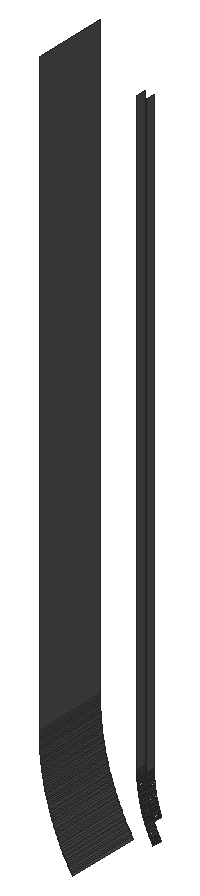
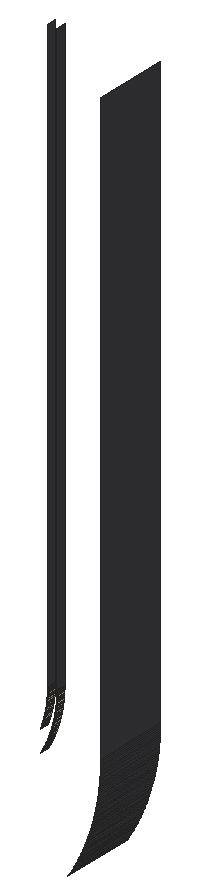
# SketchUp Ruby script. Lengths in inches.
U = 1.inch
M = Sketchup.active_model
def pt(a) = Geom::Point3d.new(a.map { |v| v * U })
def face(e, loops, mat)
  f = e.add_face(loops[0].map { |a| pt(a) })
  loops[1..].each { |l| e.add_face(l.map { |a| pt(a) }).erase! }
  f.material = f.back_material = mat if mat
  f
end
# faces: each face lists its corners as indices into pts; further lists are holes
def faces(e, pts, list, mat = nil) = list.each { |f| face(e, (f[0].is_a?(Array) ? f : [f]).map { |l| l.map { |i| pts[i] } }, mat) }
# xy, xz, yz: faces in a plane at the given z, y or x. An outline is a flat list of corners, or four numbers for a rectangle; further outlines are holes
def ring(l) = l.size == 4 ? [[l[0], l[1]], [l[2], l[1]], [l[2], l[3]], [l[0], l[3]]] : l.each_slice(2).to_a
def flat(e, list, mat, &to3) = list.each { |f| face(e, (f[0].is_a?(Array) ? f : [f]).map { |l| ring(l).map { |u, v| to3.(u, v) } }, mat) }
def xy(e, z, list, mat = nil) = flat(e, list, mat) { |x, y| [x, y, z] }
def xz(e, y, list, mat = nil) = flat(e, list, mat) { |x, z| [x, y, z] }
def yz(e, x, list, mat = nil) = flat(e, list, mat) { |y, z| [x, y, z] }
def lines(e, pts, list) = list.each { |a, b| e.add_line(pt(pts[a]), pt(pts[b])) }
# prism: a flat outline (further loops are holes) pulled along v
def prism(e, loops, v, mat = nil)
  f = face(e, loops, mat); d = Geom::Vector3d.new(v.map { |x| x * U })
  f.pushpull(f.normal.samedirection?(d) ? d.length : -d.length)
end
def box(e, o, s, mat = nil) = prism(e, [[o, [o[0] + s[0], o[1], o[2]], [o[0] + s[0], o[1] + s[1], o[2]], [o[0], o[1] + s[1], o[2]]]], [0, 0, s[2]], mat)
def at(x, y, z, deg = 0) = Geom::Transformation.translation(pt([x, y, z])) * Geom::Transformation.rotation(ORIGIN, Z_AXIS, deg.degrees)
def axes(o, x, y, z) = Geom::Transformation.new([*x, 0, *y, 0, *z, 0, *pt(o).to_a, 1])
def part(name) = M.definitions.add(name)
# library, detail: a bought-in or finely detailed component or shape, given as its bounding box
def library(name, o, s) = part(name).tap { |d| box(d.entities, o, s) }
def detail(e, o, s) = box(e.add_group.entities, o, s)
def put(e, d, t, mat = nil) = e.add_instance(d, t).tap { |i| i.material = mat if mat }
def group(e, t, mat = nil) = e.add_group.tap { |g| g.transformation = t; g.material = mat if mat }.entities
root = M.entities
M.materials.add("1432 AP 8245 TAR ROAD").color = [71, 72, 75]
M.materials.add("Outer Light").color = [251, 217, 152]
yz(root,243,[[95.37,464.23,107.37,464.51],[95.37,464.51,107.37,464.79],[95.37,464.79,107.37,560.79]],"1432 AP 8245 TAR ROAD")
yz(root,258.5,[[95.37,464.47,96.87,464.63],[95.37,464.63,96.87,464.79],[95.37,464.79,96.87,560.79]],"1432 AP 8245 TAR ROAD")
yz(root,258.5,[[95.37,464.47,96.87,464.63],[95.37,464.63,96.87,464.79],[95.37,464.79,96.87,560.79]],"Outer Light")
yz(root,258.51,[[95.37,464.15,96.87,464.31]],"1432 AP 8245 TAR ROAD")
yz(root,258.51,[[95.37,464.15,96.87,464.31]],"Outer Light")
yz(root,258.52,[[95.37,463.83,96.87,463.99]],"1432 AP 8245 TAR ROAD")
yz(root,258.52,[[95.37,463.83,96.87,463.99]],"Outer Light")
yz(root,260,[[95.37,464.49,96.87,464.64],[95.37,464.64,96.87,464.79],[95.37,464.79,96.87,560.79]],"1432 AP 8245 TAR ROAD")
yz(root,260,[[95.37,464.49,96.87,464.64],[95.37,464.64,96.87,464.79],[95.37,464.79,96.87,560.79]],"Outer Light")
yz(root,260.01,[[95.37,464.05,96.87,464.2],[95.37,464.2,96.87,464.34]],"1432 AP 8245 TAR ROAD")
yz(root,260.01,[[95.37,464.05,96.87,464.2],[95.37,464.2,96.87,464.34]],"Outer Light")
p = [[248.16,107.37,446.22],[248.3,107.37,445.98],[248.3,95.37,445.98],[248.16,95.37,446.22],[248.01,107.37,446.47],[248.01,95.37,446.47],
  [247.87,107.37,446.71],[247.87,95.37,446.71],[247.73,107.37,446.96],[247.73,95.37,446.96],[247.59,107.37,447.2],[247.59,95.37,447.2],
  [247.45,107.37,447.45],[247.45,95.37,447.45],[247.32,107.37,447.7],[247.32,95.37,447.7],[247.18,107.37,447.95],[247.18,95.37,447.95],
  [247.05,107.37,448.2],[247.05,95.37,448.2],[246.92,107.37,448.45],[246.92,95.37,448.45],[246.8,107.37,448.7],[246.8,95.37,448.7],
  [246.67,107.37,448.95],[246.67,95.37,448.95],[246.55,107.37,449.21],[246.55,95.37,449.21],[246.43,107.37,449.46],[246.43,95.37,449.46],
  [246.31,107.37,449.72],[246.31,95.37,449.72],[246.1875,107.37,449.98],[246.1875,95.37,449.98],[246.07,107.37,450.24],[246.07,95.37,450.24],
  [245.96,107.37,450.49],[245.96,95.37,450.49],[245.85,107.37,450.75],[245.85,95.37,450.75],[245.74,107.37,451.02],[245.74,95.37,451.02],
  [245.63,107.37,451.28],[245.63,95.37,451.28],[245.53,107.37,451.54],[245.53,95.37,451.54],[245.42,107.37,451.8],[245.42,95.37,451.8],
  [245.32,107.37,452.07],[245.32,95.37,452.07],[245.23,107.37,452.33],[245.23,95.37,452.33],[245.13,107.37,452.6],[245.13,95.37,452.6],
  [245.03,107.37,452.86],[245.03,95.37,452.86],[244.94,107.37,453.13],[244.94,95.37,453.13],[244.85,107.37,453.4],[244.85,95.37,453.4],
  [244.76,107.37,453.67],[244.76,95.37,453.67],[244.68,107.37,453.9375],[244.68,95.37,453.9375],[244.59,107.37,454.21],[244.59,95.37,454.21],
  [244.51,107.37,454.48],[244.51,95.37,454.48],[244.43,107.37,454.75],[244.43,95.37,454.75],[244.35,107.37,455.02],[244.35,95.37,455.02],
  [261.04,95.37,454.92],[261.11,95.37,454.78],[261.11,96.87,454.78],[261.04,96.87,454.92],[261.04,96.87,454.92],[261.11,96.87,454.78],
  [261.11,95.37,454.78],[261.04,95.37,454.92],[260.96,95.37,455.06],[260.96,96.87,455.06],[260.96,96.87,455.06],[260.96,95.37,455.06],
  [244.28,107.37,455.29],[244.28,95.37,455.29],[260.88,95.37,455.2],[260.88,96.87,455.2],[260.88,96.87,455.2],[260.88,95.37,455.2],
  [260.81,95.37,455.34],[260.81,96.87,455.34],[260.81,96.87,455.34],[260.81,95.37,455.34],[244.2,107.37,455.57],[244.2,95.37,455.57],
  [260.73,95.37,455.49],[260.73,96.87,455.49],[260.73,96.87,455.49],[260.73,95.37,455.49],[260.66,95.37,455.63],[260.66,96.87,455.63],
  [260.66,96.87,455.63],[260.66,95.37,455.63],[244.13,107.37,455.84],[244.13,95.37,455.84],[260.59,95.37,455.77],[260.59,96.87,455.77],
  [260.59,96.87,455.77],[260.59,95.37,455.77],[244.0625,107.37,456.11],[244.0625,95.37,456.11],[260.52,95.37,455.92],[260.52,96.87,455.92],
  [260.52,96.87,455.92],[260.52,95.37,455.92],[260.45,95.37,456.0625],[260.45,96.87,456.0625],[260.45,96.87,456.0625],[260.45,95.37,456.0625],
  [243.99,107.37,456.39],[243.99,95.37,456.39],[260.38,95.37,456.21],[260.38,96.87,456.21],[260.38,96.87,456.21],[260.38,95.37,456.21],
  [260.32,95.37,456.36],[260.32,96.87,456.36],[260.32,96.87,456.36],[260.32,95.37,456.36],[243.93,107.37,456.66],[243.93,95.37,456.66],
  [260.25,95.37,456.5],[260.25,96.87,456.5],[260.25,96.87,456.5],[260.25,95.37,456.5],[260.1875,95.37,456.65],[260.1875,96.87,456.65],
  [260.1875,96.87,456.65],[260.1875,95.37,456.65],[243.87,107.37,456.9375],[243.87,95.37,456.9375],[260.12,95.37,456.8],[260.12,96.87,456.8],
  [260.12,96.87,456.8],[260.12,95.37,456.8],[260.06,95.37,456.95],[260.06,96.87,456.95],[260.06,96.87,456.95],[260.06,95.37,456.95],
  [243.81,107.37,457.22],[243.81,95.37,457.22],[260,95.37,457.1],[260,96.87,457.1],[260,96.87,457.1],[260,95.37,457.1],
  [259.94,95.37,457.25],[259.94,96.87,457.25],[259.94,96.87,457.25],[259.94,95.37,457.25],[243.75,107.37,457.49],[243.75,95.37,457.49],
  [259.88,95.37,457.4],[259.88,96.87,457.4],[259.88,96.87,457.4],[259.88,95.37,457.4],[259.82,95.37,457.55],[259.82,96.87,457.55],
  [259.82,96.87,457.55],[259.82,95.37,457.55],[243.69,107.37,457.77],[243.69,95.37,457.77],[259.77,95.37,457.7],[259.77,96.87,457.7],
  [259.77,96.87,457.7],[259.77,95.37,457.7],[259.71,95.37,457.85],[259.71,96.87,457.85],[259.71,96.87,457.85],[259.71,95.37,457.85],
  [243.64,107.37,458.05],[243.64,95.37,458.05],[259.66,95.37,458],[259.66,96.87,458],[259.66,96.87,458],[259.66,95.37,458],
  [243.59,107.37,458.32],[243.59,95.37,458.32],[259.61,95.37,458.15],[259.61,96.87,458.15],[259.61,96.87,458.15],[259.61,95.37,458.15],
  [259.55,95.37,458.3],[259.55,96.87,458.3],[259.55,96.87,458.3],[259.55,95.37,458.3],[261.17,95.37,458.22],[261.125,95.37,458.36],
  [261.125,96.87,458.36],[261.17,96.87,458.22],[243.54,107.37,458.6],[243.54,95.37,458.6],[259.5,95.37,458.46],[259.5,96.87,458.46],
  [259.5,96.87,458.46],[259.5,95.37,458.46],[261.07,95.37,458.5],[261.07,96.87,458.5],[261.125,96.87,458.36],[261.07,96.87,458.5],
  [261.07,95.37,458.5],[261.125,95.37,458.36],[259.45,95.37,458.61],[259.45,96.87,458.61],[259.45,96.87,458.61],[259.45,95.37,458.61],
  [261.02,95.37,458.64],[261.02,96.87,458.64],[261.02,96.87,458.64],[261.02,95.37,458.64],[243.49,107.37,458.88],[243.49,95.37,458.88],
  [259.41,95.37,458.76],[259.41,96.87,458.76],[259.41,96.87,458.76],[259.41,95.37,458.76],[260.98,95.37,458.78],[260.98,96.87,458.78],
  [260.98,96.87,458.78],[260.98,95.37,458.78],[259.36,95.37,458.92],[259.36,96.87,458.92],[259.36,96.87,458.92],[259.36,95.37,458.92],
  [260.93,95.37,458.92],[260.93,96.87,458.92],[260.93,96.87,458.92],[260.93,95.37,458.92],[243.44,107.37,459.16],[243.44,95.37,459.16],
  [259.3125,95.37,459.07],[259.3125,96.87,459.07],[259.3125,96.87,459.07],[259.3125,95.37,459.07],[260.88,95.37,459.0625],[260.88,96.87,459.0625],
  [260.88,96.87,459.0625],[260.88,95.37,459.0625],[259.27,95.37,459.23],[259.27,96.87,459.23],[259.27,96.87,459.23],[259.27,95.37,459.23],
  [260.84,95.37,459.21],[260.84,96.87,459.21],[260.84,96.87,459.21],[260.84,95.37,459.21],[243.4,107.37,459.44],[243.4,95.37,459.44],
  [259.23,95.37,459.38],[259.23,96.87,459.38],[259.23,96.87,459.38],[259.23,95.37,459.38],[260.8,95.37,459.35],[260.8,96.87,459.35],
  [260.8,96.87,459.35],[260.8,95.37,459.35],[260.75,95.37,459.49],[260.75,96.87,459.49],[260.75,96.87,459.49],[260.75,95.37,459.49],
  [243.36,107.37,459.72],[243.36,95.37,459.72],[259.18,95.37,459.54],[259.18,96.87,459.54],[259.18,96.87,459.54],[259.18,95.37,459.54],
  [259.14,95.37,459.69],[259.14,96.87,459.69],[259.14,96.87,459.69],[259.14,95.37,459.69],[260.71,95.37,459.63],[260.71,96.87,459.63],
  [260.71,96.87,459.63],[260.71,95.37,459.63],[260.67,95.37,459.78],[260.67,96.87,459.78],[260.67,96.87,459.78],[260.67,95.37,459.78],
  [243.32,107.37,460],[243.32,95.37,460],[259.1,95.37,459.85],[259.1,96.87,459.85],[259.1,96.87,459.85],[259.1,95.37,459.85],
  [260.63,95.37,459.92],[260.63,96.87,459.92],[260.63,96.87,459.92],[260.63,95.37,459.92],[259.07,95.37,460.01],[259.07,96.87,460.01],
  [259.07,96.87,460.01],[259.07,95.37,460.01],[260.6,95.37,460.07],[260.6,96.87,460.07],[260.6,96.87,460.07],[260.6,95.37,460.07],
  [243.28,107.37,460.28],[243.28,95.37,460.28],[259.03,95.37,460.16],[259.03,96.87,460.16],[259.03,96.87,460.16],[259.03,95.37,460.16],
  [260.56,95.37,460.21],[260.56,96.87,460.21],[260.56,96.87,460.21],[260.56,95.37,460.21],[258.99,95.37,460.32],[258.99,96.87,460.32],
  [258.99,96.87,460.32],[258.99,95.37,460.32],[260.52,95.37,460.36],[260.52,96.87,460.36],[260.52,96.87,460.36],[260.52,95.37,460.36],
  [243.25,107.37,460.5625],[243.25,95.37,460.5625],[258.96,95.37,460.48],[258.96,96.87,460.48],[258.96,96.87,460.48],[258.96,95.37,460.48],
  [260.49,95.37,460.5],[260.49,96.87,460.5],[260.49,96.87,460.5],[260.49,95.37,460.5],[258.93,95.37,460.63],[258.93,96.87,460.63],
  [258.93,96.87,460.63],[258.93,95.37,460.63],[260.46,95.37,460.65],[260.46,96.87,460.65],[260.46,96.87,460.65],[260.46,95.37,460.65],
  [243.22,107.37,460.84],[243.22,95.37,460.84],[258.89,95.37,460.79],[258.89,96.87,460.79],[258.89,96.87,460.79],[258.89,95.37,460.79],
  [260.43,95.37,460.79],[260.43,96.87,460.79],[260.43,96.87,460.79],[260.43,95.37,460.79],[243.1875,107.37,461.12],[243.1875,95.37,461.12],
  [258.86,95.37,460.95],[258.86,96.87,460.95],[258.86,96.87,460.95],[258.86,95.37,460.95],[260.39,95.37,460.9375],[260.39,96.87,460.9375],
  [260.39,96.87,460.9375],[260.39,95.37,460.9375],[260.37,95.37,461.09],[260.37,96.87,461.09],[260.37,96.87,461.09],[260.37,95.37,461.09],
  [258.83,95.37,461.11],[258.83,96.87,461.11],[258.83,96.87,461.11],[258.83,95.37,461.11],[243.16,107.37,461.4],[243.16,95.37,461.4],
  [258.81,95.37,461.27],[258.81,96.87,461.27],[258.81,96.87,461.27],[258.81,95.37,461.27],[260.34,95.37,461.23],[260.34,96.87,461.23],
  [260.34,96.87,461.23],[260.34,95.37,461.23],[260.31,95.37,461.38],[260.31,96.87,461.38],[260.31,96.87,461.38],[260.31,95.37,461.38],
  [258.78,95.37,461.43],[258.78,96.87,461.43],[258.78,96.87,461.43],[258.78,95.37,461.43],[243.13,107.37,461.6875],[243.13,95.37,461.6875],
  [258.75,95.37,461.59],[258.75,96.87,461.59],[258.75,96.87,461.59],[258.75,95.37,461.59],[260.28,95.37,461.53],[260.28,96.87,461.53],
  [260.28,96.87,461.53],[260.28,95.37,461.53],[260.26,95.37,461.67],[260.26,96.87,461.67],[260.26,96.87,461.67],[260.26,95.37,461.67],
  [258.73,95.37,461.74],[258.73,96.87,461.74],[258.73,96.87,461.74],[258.73,95.37,461.74],[243.11,107.37,461.97],[243.11,95.37,461.97],
  [258.7,95.37,461.9],[258.7,96.87,461.9],[258.7,96.87,461.9],[258.7,95.37,461.9],[260.23,95.37,461.82],[260.23,96.87,461.82],
  [260.23,96.87,461.82],[260.23,95.37,461.82],[260.21,95.37,461.97],[260.21,96.87,461.97],[260.21,96.87,461.97],[260.21,95.37,461.97],
  [258.68,95.37,462.0625],[258.68,96.87,462.0625],[258.68,96.87,462.0625],[258.68,95.37,462.0625],[243.09,107.37,462.25],[243.09,95.37,462.25],
  [260.19,95.37,462.11],[260.19,96.87,462.11],[260.19,96.87,462.11],[260.19,95.37,462.11],[258.66,95.37,462.22],[258.66,96.87,462.22],
  [258.66,96.87,462.22],[258.66,95.37,462.22],[260.17,95.37,462.26],[260.17,96.87,462.26],[260.17,96.87,462.26],[260.17,95.37,462.26],
  [243.07,107.37,462.53],[243.07,95.37,462.53],[258.64,95.37,462.38],[258.64,96.87,462.38],[258.64,96.87,462.38],[258.64,95.37,462.38],
  [260.15,95.37,462.41],[260.15,96.87,462.41],[260.15,96.87,462.41],[260.15,95.37,462.41],[258.625,95.37,462.54],[258.625,96.87,462.54],
  [258.625,96.87,462.54],[258.625,95.37,462.54],[260.13,95.37,462.56],[260.13,96.87,462.56],[260.13,96.87,462.56],[260.13,95.37,462.56],
  [243.05,107.37,462.8125],[243.05,95.37,462.8125],[258.61,95.37,462.7],[258.61,96.87,462.7],[258.61,96.87,462.7],[258.61,95.37,462.7],
  [260.11,95.37,462.71],[260.11,96.87,462.71],[260.11,96.87,462.71],[260.11,95.37,462.71],[258.59,95.37,462.86],[258.59,96.87,462.86],
  [258.59,96.87,462.86],[258.59,95.37,462.86],[260.1,95.37,462.86],[260.1,96.87,462.86],[260.1,96.87,462.86],[260.1,95.37,462.86],
  [243.04,107.37,463.1],[243.04,95.37,463.1],[258.58,95.37,463.02],[258.58,96.87,463.02],[258.58,96.87,463.02],[258.58,95.37,463.02],
  [260.08,95.37,463],[260.08,96.87,463],[260.08,96.87,463],[260.08,95.37,463],[258.5625,95.37,463.18],[258.5625,96.87,463.18],
  [258.5625,96.87,463.18],[258.5625,95.37,463.18],[260.07,95.37,463.15],[260.07,96.87,463.15],[260.07,96.87,463.15],[260.07,95.37,463.15],
  [243.03,107.37,463.38],[243.03,95.37,463.38],[258.55,95.37,463.34],[258.55,96.87,463.34],[258.55,96.87,463.34],[258.55,95.37,463.34],
  [260.06,95.37,463.3],[260.06,96.87,463.3],[260.06,96.87,463.3],[260.06,95.37,463.3],[258.54,95.37,463.5],[258.54,96.87,463.5],
  [258.54,96.87,463.5],[258.54,95.37,463.5],[260.05,95.37,463.45],[260.05,96.87,463.45],[260.05,96.87,463.45],[260.05,95.37,463.45],
  [243.02,107.37,463.66],[243.02,95.37,463.66],[258.53,95.37,463.67],[258.53,96.87,463.67],[258.53,96.87,463.67],[258.53,95.37,463.67],
  [260.04,95.37,463.6],[260.04,96.87,463.6],[260.04,96.87,463.6],[260.04,95.37,463.6],[260.03,95.37,463.75],[260.03,96.87,463.75],
  [260.03,96.87,463.75],[260.03,95.37,463.75],[243.01,107.37,463.94],[243.01,95.37,463.94],[258.52,95.37,463.83],[258.52,96.87,463.83],
  [258.52,96.87,463.83],[258.52,95.37,463.83],[260.02,95.37,463.9],[260.02,96.87,463.9],[260.02,96.87,463.9],[260.02,95.37,463.9],
  [243,107.37,464.23],[243,95.37,464.23],[260.01,95.37,464.05],[260.01,96.87,464.05],[260.01,96.87,464.05],[260.01,95.37,464.05],
  [258.51,95.37,464.15],[258.52,95.37,463.99],[258.52,96.87,463.99],[258.51,96.87,464.15],[258.51,96.87,464.15],[258.52,96.87,463.99],
  [258.52,95.37,463.99],[258.51,95.37,464.15],[258.5,95.37,464.47],[258.51,95.37,464.31],[258.51,96.87,464.31],[258.5,96.87,464.47],
  [258.5,96.87,464.47],[258.51,96.87,464.31],[258.51,95.37,464.31],[258.5,95.37,464.47],[260.01,95.37,464.34],[260,95.37,464.49],
  [260,96.87,464.49],[260.01,96.87,464.34],[260.01,96.87,464.34],[260,96.87,464.49],[260,95.37,464.49],[260.01,95.37,464.34]]
faces(root,p,[[0,1,2,3],[4,0,3,5],[6,4,5,7],[8,6,7,9],[10,8,9,11],[12,10,11,13],[14,12,13,15],[16,14,15,17],
  [18,16,17,19],[20,18,19,21],[22,20,21,23],[24,22,23,25],[26,24,25,27],[28,26,27,29],[30,28,29,31],[32,30,31,33],
  [34,32,33,35],[36,34,35,37],[38,36,37,39],[40,38,39,41],[42,40,41,43],[44,42,43,45],[46,44,45,47],[48,46,47,49],
  [50,48,49,51],[52,50,51,53],[54,52,53,55],[56,54,55,57],[58,56,57,59],[60,58,59,61],[62,60,61,63],[64,62,63,65],
  [66,64,65,67],[68,66,67,69],[70,68,69,71],[72,73,74,75],[80,72,75,81],[84,70,71,85],[86,80,81,87],[90,86,87,91],
  [94,84,85,95],[96,90,91,97],[100,96,97,101],[104,94,95,105],[106,100,101,107],[110,104,105,111],[112,106,107,113],[116,112,113,117],
  [120,110,111,121],[122,116,117,123],[126,122,123,127],[130,120,121,131],[132,126,127,133],[136,132,133,137],[140,130,131,141],[142,136,137,143],
  [146,142,143,147],[150,140,141,151],[152,146,147,153],[156,152,153,157],[160,150,151,161],[162,156,157,163],[166,162,163,167],[170,160,161,171],
  [172,166,167,173],[176,172,173,177],[180,170,171,181],[182,176,177,183],[186,180,181,187],[188,182,183,189],[192,188,189,193],[196,197,198,199],
  [200,186,187,201],[202,192,193,203],[197,206,207,198],[212,202,203,213],[206,216,217,207],[220,200,201,221],[222,212,213,223],[216,226,227,217],
  [230,222,223,231],[226,234,235,227],[238,220,221,239],[240,230,231,241],[234,244,245,235],[248,240,241,249],[244,252,253,245],[256,238,239,257],
  [258,248,249,259],[252,262,263,253],[262,266,267,263],[270,256,257,271],[272,258,259,273],[276,272,273,277],[266,280,281,267],[280,284,285,281],
  [288,270,271,289],[290,276,277,291],[284,294,295,285],[298,290,291,299],[294,302,303,295],[306,288,289,307],[308,298,299,309],[302,312,313,303],
  [316,308,309,317],[312,320,321,313],[324,306,307,325],[326,316,317,327],[320,330,331,321],[334,326,327,335],[330,338,339,331],[342,324,325,343],
  [344,334,335,345],[338,348,349,339],[352,342,343,353],[354,344,345,355],[348,358,359,349],[358,362,363,359],[366,354,355,367],[370,352,353,371],
  [372,366,367,373],[362,376,377,363],[376,380,381,377],[384,372,373,385],[388,370,371,389],[390,384,385,391],[380,394,395,381],[394,398,399,395],
  [402,390,391,403],[406,388,389,407],[408,402,403,409],[398,412,413,399],[412,416,417,413],[420,408,409,421],[424,406,407,425],[416,426,427,417],
  [430,420,421,431],[426,434,435,427],[438,424,425,439],[440,430,431,441],[434,444,445,435],[448,440,441,449],[444,452,453,445],[456,438,439,457],
  [458,448,449,459],[452,462,463,453],[466,458,459,467],[462,470,471,463],[474,456,457,475],[476,466,467,477],[470,480,481,471],[484,476,477,485],
  [480,488,489,481],[492,474,475,493],[494,484,485,495],[488,498,499,489],[502,494,495,503],[498,506,507,499],[510,492,493,511],[512,502,503,513],
  [506,516,517,507],[516,520,521,517],[524,510,511,525],[526,512,513,527],[520,530,531,521],[534,524,525,535],[530,536,537,531],[540,541,542,543],
  [548,549,550,551],[556,557,558,559]],"1432 AP 8245 TAR ROAD")
faces(root,p,[[76,77,78,79],[82,76,79,83],[88,82,83,89],[92,88,89,93],[98,92,93,99],[102,98,99,103],[108,102,103,109],[114,108,109,115],
  [118,114,115,119],[124,118,119,125],[128,124,125,129],[134,128,129,135],[138,134,135,139],[144,138,139,145],[148,144,145,149],[154,148,149,155],
  [158,154,155,159],[164,158,159,165],[168,164,165,169],[174,168,169,175],[178,174,175,179],[184,178,179,185],[190,184,185,191],[194,190,191,195],
  [204,194,195,205],[208,209,210,211],[214,204,205,215],[209,218,219,210],[224,214,215,225],[218,228,229,219],[232,224,225,233],[228,236,237,229],
  [242,232,233,243],[236,246,247,237],[250,242,243,251],[246,254,255,247],[260,250,251,261],[254,264,265,255],[264,268,269,265],[274,260,261,275],
  [278,274,275,279],[268,282,283,269],[282,286,287,283],[292,278,279,293],[286,296,297,287],[300,292,293,301],[296,304,305,297],[310,300,301,311],
  [304,314,315,305],[318,310,311,319],[314,322,323,315],[328,318,319,329],[322,332,333,323],[336,328,329,337],[332,340,341,333],[346,336,337,347],
  [340,350,351,341],[356,346,347,357],[350,360,361,351],[360,364,365,361],[368,356,357,369],[374,368,369,375],[364,378,379,365],[378,382,383,379],
  [386,374,375,387],[392,386,387,393],[382,396,397,383],[396,400,401,397],[404,392,393,405],[410,404,405,411],[400,414,415,401],[414,418,419,415],
  [422,410,411,423],[418,428,429,419],[432,422,423,433],[428,436,437,429],[442,432,433,443],[436,446,447,437],[450,442,443,451],[446,454,455,447],
  [460,450,451,461],[454,464,465,455],[468,460,461,469],[464,472,473,465],[478,468,469,479],[472,482,483,473],[486,478,479,487],[482,490,491,483],
  [496,486,487,497],[490,500,501,491],[504,496,497,505],[500,508,509,501],[514,504,505,515],[508,518,519,509],[518,522,523,519],[528,514,515,529],
  [522,532,533,523],[532,538,539,533],[544,545,546,547],[552,553,554,555],[560,561,562,563]],"Outer Light")
